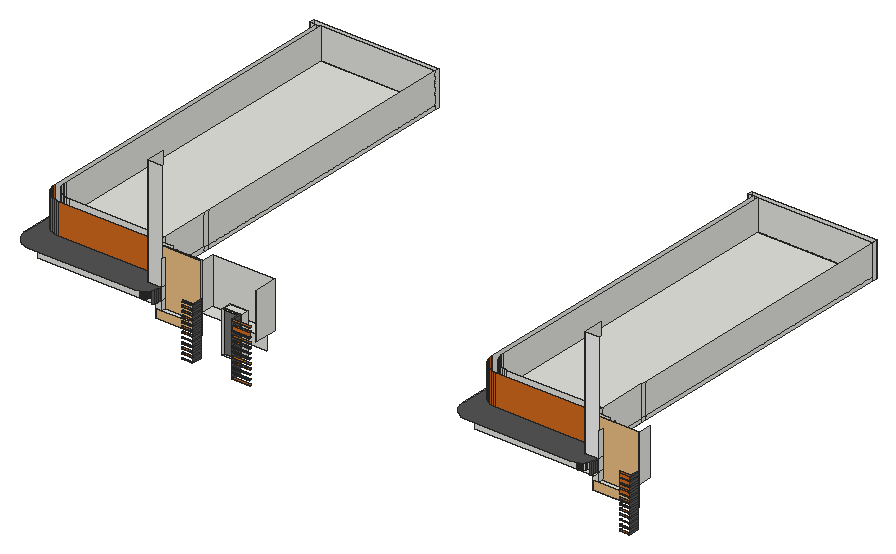
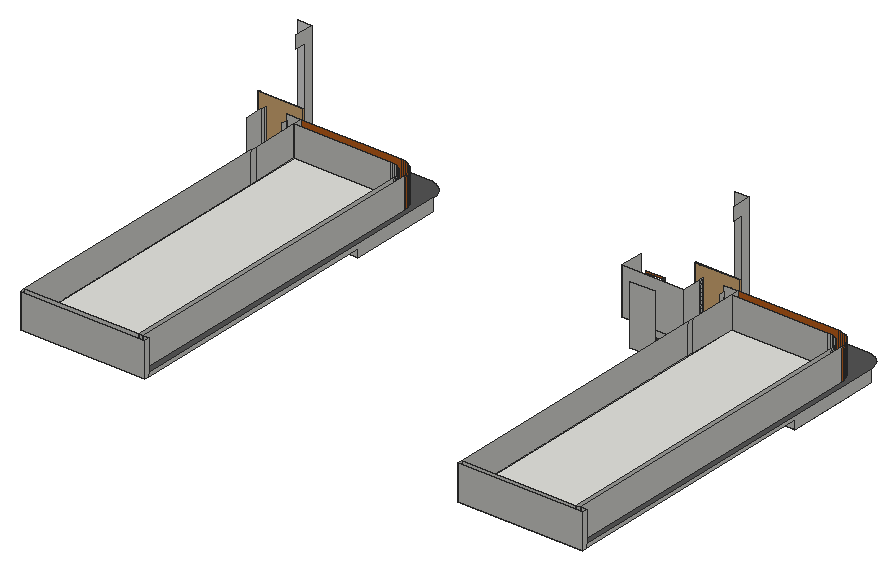
# SketchUp Ruby script. Lengths in inches.
U = 1.inch
M = Sketchup.active_model
def pt(a) = Geom::Point3d.new(a.map { |v| v * U })
def face(e, loops, mat)
  f = e.add_face(loops[0].map { |a| pt(a) })
  loops[1..].each { |l| e.add_face(l.map { |a| pt(a) }).erase! }
  f.material = f.back_material = mat if mat
  f
end
# faces: each face lists its corners as indices into pts; further lists are holes
def faces(e, pts, list, mat = nil) = list.each { |f| face(e, (f[0].is_a?(Array) ? f : [f]).map { |l| l.map { |i| pts[i] } }, mat) }
# xy, xz, yz: faces in a plane at the given z, y or x. An outline is a flat list of corners, or four numbers for a rectangle; further outlines are holes
def ring(l) = l.size == 4 ? [[l[0], l[1]], [l[2], l[1]], [l[2], l[3]], [l[0], l[3]]] : l.each_slice(2).to_a
def flat(e, list, mat, &to3) = list.each { |f| face(e, (f[0].is_a?(Array) ? f : [f]).map { |l| ring(l).map { |u, v| to3.(u, v) } }, mat) }
def xy(e, z, list, mat = nil) = flat(e, list, mat) { |x, y| [x, y, z] }
def xz(e, y, list, mat = nil) = flat(e, list, mat) { |x, z| [x, y, z] }
def yz(e, x, list, mat = nil) = flat(e, list, mat) { |y, z| [x, y, z] }
def lines(e, pts, list) = list.each { |a, b| e.add_line(pt(pts[a]), pt(pts[b])) }
# prism: a flat outline (further loops are holes) pulled along v
def prism(e, loops, v, mat = nil)
  f = face(e, loops, mat); d = Geom::Vector3d.new(v.map { |x| x * U })
  f.pushpull(f.normal.samedirection?(d) ? d.length : -d.length)
end
def box(e, o, s, mat = nil) = prism(e, [[o, [o[0] + s[0], o[1], o[2]], [o[0] + s[0], o[1] + s[1], o[2]], [o[0], o[1] + s[1], o[2]]]], [0, 0, s[2]], mat)
def at(x, y, z, deg = 0) = Geom::Transformation.translation(pt([x, y, z])) * Geom::Transformation.rotation(ORIGIN, Z_AXIS, deg.degrees)
def axes(o, x, y, z) = Geom::Transformation.new([*x, 0, *y, 0, *z, 0, *pt(o).to_a, 1])
def part(name) = M.definitions.add(name)
# library, detail: a bought-in or finely detailed component or shape, given as its bounding box
def library(name, o, s) = part(name).tap { |d| box(d.entities, o, s) }
def detail(e, o, s) = box(e.add_group.entities, o, s)
def put(e, d, t, mat = nil) = e.add_instance(d, t).tap { |i| i.material = mat if mat }
def group(e, t, mat = nil) = e.add_group.tap { |g| g.transformation = t; g.material = mat if mat }.entities
root = M.entities
M.materials.add("[0039_DarkOrange]").color = [219, 120, 0]
M.materials.add("[0041_Chocolate]").color = [210, 105, 30]
M.materials.add("[0129_WhiteSmoke]").color = [245, 245, 245]
M.materials.add("[Color M06]").color = [84, 84, 84]
M.materials.add("[Translucent Glass Gray]").color = [0, 0, 0]
M.materials["[Translucent Glass Gray]"].alpha = 0.5
c1 = library("1",[3.97,34.78,0],[101.43,33.99,0.79])
xy(root,180.58,[[820.52,971.36,835.91,972.36],[895.48,971.36,921.96,972.36],[1476.02,971.36,1491.41,972.36]],"[0041_Chocolate]")
xy(root,182.6875,[[820.52,971.36,835.91,972.36],[895.48,971.36,921.96,972.36],[1476.02,971.36,1491.41,972.36]],"[0041_Chocolate]")
xy(root,187.64,[[820.52,971.36,835.91,972.36],[895.48,971.36,921.96,972.36],[1476.02,971.36,1491.41,972.36]],"[0041_Chocolate]")
xy(root,189.75,[[820.52,971.36,835.91,972.36],[895.48,971.36,921.96,972.36],[1476.02,971.36,1491.41,972.36]],"[0041_Chocolate]")
xy(root,194.7,[[820.52,971.36,835.91,972.36],[895.48,971.36,921.96,972.36],[1476.02,971.36,1491.41,972.36]],"[0041_Chocolate]")
xy(root,196.8125,[[895.48,971.36,921.96,972.36]],"[0039_DarkOrange]")
xy(root,196.8125,[[820.52,971.36,835.91,972.36],[1476.02,971.36,1491.41,972.36]],"[0041_Chocolate]")
xy(root,196.89,[[868.14,986.55,894.83,989.22],[868.14,990.13,894.83,1001.8]])
xy(root,201.77,[[895.48,971.36,921.96,972.36]],"[0039_DarkOrange]")
xy(root,201.77,[[820.52,971.36,835.91,972.36],[1476.02,971.36,1491.41,972.36]],"[0041_Chocolate]")
xy(root,203.875,[[895.48,971.36,921.96,972.36]],"[0039_DarkOrange]")
xy(root,203.875,[[820.52,971.36,835.91,972.36],[1476.02,971.36,1491.41,972.36]],"[0041_Chocolate]")
xy(root,208.83,[[895.48,971.36,921.96,972.36]],"[0039_DarkOrange]")
xy(root,208.83,[[820.52,971.36,835.91,972.36],[1476.02,971.36,1491.41,972.36]],"[0041_Chocolate]")
xy(root,210.9375,[[895.48,971.36,921.96,972.36]],"[0039_DarkOrange]")
xy(root,210.9375,[[820.52,971.36,835.91,972.36],[1476.02,971.36,1491.41,972.36]],"[0041_Chocolate]")
xy(root,215.89,[[895.48,971.36,921.96,972.36]],"[0039_DarkOrange]")
xy(root,215.89,[[820.52,971.36,835.91,972.36],[1476.02,971.36,1491.41,972.36]],"[0041_Chocolate]")
xy(root,218,[[895.48,971.36,921.96,972.36]],"[0039_DarkOrange]")
xy(root,218,[[820.52,971.36,835.91,972.36],[1476.02,971.36,1491.41,972.36]],"[0041_Chocolate]")
xy(root,222.95,[[895.48,971.36,921.96,972.36]],"[0039_DarkOrange]")
xy(root,222.95,[[820.52,971.36,835.91,972.36],[1476.02,971.36,1491.41,972.36]],"[0041_Chocolate]")
xy(root,225.0625,[[895.48,971.36,921.96,972.36]],"[0039_DarkOrange]")
xy(root,225.0625,[[820.52,971.36,835.91,972.36],[1476.02,971.36,1491.41,972.36]],"[0041_Chocolate]")
xy(root,226.8,[[770.9,983.34,780.56,996.48],[780.56,983.34,820.52,1028.46],[1426.4,983.34,1436.06,996.48],[1436.06,983.34,1476.02,1028.46],[820.52,1008.21,913.34,1028.46]])
xy(root,227.53,[[700.74,1086.875,747.92,1094.0625],[1356.24,1086.875,1403.42,1094.0625]])
xy(root,230.02,[[895.48,971.36,921.96,972.36]],"[0039_DarkOrange]")
xy(root,230.02,[[820.52,971.36,835.91,972.36],[1476.02,971.36,1491.41,972.36]],"[0041_Chocolate]")
xy(root,232.125,[[895.48,971.36,921.96,972.36]],"[0039_DarkOrange]")
xy(root,232.125,[[820.52,971.36,835.91,972.36],[1476.02,971.36,1491.41,972.36]],"[0041_Chocolate]")
xy(root,237.08,[[895.48,971.36,921.96,972.36]],"[0039_DarkOrange]")
xy(root,237.08,[[820.52,971.36,835.91,972.36],[1476.02,971.36,1491.41,972.36]],"[0041_Chocolate]")
xy(root,239.1875,[[820.52,971.36,835.91,972.36],[895.48,971.36,921.96,972.36],[1476.02,971.36,1491.41,972.36]],"[0041_Chocolate]")
xy(root,240.16,[[756.44,972.36,757.68,972.44,758.91,972.69,759.32,972.82,759.32,972.36],[759.32,972.36,759.32,972.82,760.09,973.09,761.21,973.64,762.24,974.33,763.18,975.15,764,976.09,764.7,977.13,765.25,978.25,765.65,979.43,765.89,980.65,765.97,981.89,759.32,981.89,759.32,983.34,779.69,983.34,779.69,981.89,779.49,978.86,778.9,975.875,777.92,973,777.61,972.36],[777.61,972.36,780.56,972.36,780.56,981.89,779.69,981.89,779.49,978.86,778.9,975.875,777.92,973],[1411.94,972.36,1413.18,972.44,1414.41,972.69,1414.82,972.82,1414.82,972.36],[1414.82,972.36,1414.82,972.82,1415.59,973.09,1416.71,973.64,1417.74,974.33,1418.68,975.15,1419.5,976.09,1420.2,977.13,1420.75,978.25,1421.15,979.43,1421.39,980.65,1421.47,981.89,1414.82,981.89,1414.82,983.34,1435.19,983.34,1435.19,981.89,1434.99,978.86,1434.4,975.875,1433.42,973,1433.11,972.36],
  [1433.11,972.36,1436.06,972.36,1436.06,981.89,1435.19,981.89,1434.99,978.86,1434.4,975.875,1433.42,973],[759.32,972.82,760.09,973.09,761.21,973.64,762.24,974.33,763.18,975.15,764,976.09,764.7,977.13,765.25,978.25,765.65,979.43,765.89,980.65,765.97,981.89,759.32,981.89],[1414.82,972.82,1415.59,973.09,1416.71,973.64,1417.74,974.33,1418.68,975.15,1419.5,976.09,1420.2,977.13,1420.75,978.25,1421.15,979.43,1421.39,980.65,1421.47,981.89,1414.82,981.89],[779.69,981.89,780.56,983.34],[1435.19,981.89,1436.06,983.34],
  [759.32,983.34,779.69,1003.71],[779.69,983.34,780.56,1003.71],[1414.82,983.34,1435.19,1003.71],[1435.19,983.34,1436.06,1003.71]])
xy(root,240.16,[[572.21,1024.22,585.93,1130.875],[1227.71,1024.22,1241.43,1130.875]],"[Color M06]")
xy(root,244.14,[[820.52,971.36,835.91,972.36],[895.48,971.36,921.96,972.36],[1476.02,971.36,1491.41,972.36]],"[0041_Chocolate]")
xy(root,246.25,[[820.52,971.36,835.91,972.36],[895.48,971.36,921.96,972.36],[1476.02,971.36,1491.41,972.36]],"[0041_Chocolate]")
xy(root,251.2,[[820.52,971.36,835.91,972.36],[895.48,971.36,921.96,972.36],[1476.02,971.36,1491.41,972.36]],"[0041_Chocolate]")
xy(root,252.47,[[602.85,972.36,600.64,972.5,598.47,972.9375,596.37,973.65,594.39,974.63,592.55,975.86,590.88,977.32,589.42,978.98,588.19,980.82,587.21,982.81,586.5,984.9,586.07,987.07,585.93,989.28,585.93,1130.875,688.99,1130.875,688.99,1086.875,759.32,1086.875,759.32,981.89,765.97,981.89,765.89,980.65,765.65,979.43,765.25,978.25,764.7,977.13,764,976.09,763.18,975.15,762.24,974.33,761.21,973.64,760.09,973.09,758.91,972.69,757.68,972.44,756.44,972.36],[1258.35,972.36,1256.14,972.5,1253.97,972.9375,1251.87,973.65,1249.89,974.63,1248.05,975.86,1246.38,977.32,1244.92,978.98,1243.69,980.82,1242.71,982.81,1242,984.9,1241.57,987.07,1241.43,989.28,1241.43,1130.875,1344.49,1130.875,1344.49,1086.875,1414.82,1086.875,1414.82,981.89,1421.47,981.89,1421.39,980.65,1421.15,979.43,1420.75,978.25,1420.2,977.13,1419.5,976.09,1418.68,975.15,1417.74,974.33,1416.71,973.64,1415.59,973.09,1414.41,972.69,1413.18,972.44,1411.94,972.36],[[688.99,1086.875,759.32,1086.875,759.32,1094.0625,706.57,1094.0625,706.57,1130.875,759.32,1130.875,759.32,1521.81,572.21,1521.81,572.21,1130.875,688.99,1130.875],[577.71,1136.38,753.81,1516.3]],[[1344.49,1086.875,1414.82,1086.875,1414.82,1094.0625,1362.07,1094.0625,1362.07,1130.875,1414.82,1130.875,1414.82,1521.81,1227.71,1521.81,1227.71,1130.875,1344.49,1130.875],[1233.21,1136.38,1409.31,1516.3]],[706.57,1094.0625,759.32,1130.875],
  [1362.07,1094.0625,1414.82,1130.875],[572.21,1521.81,759.32,1529.04],[1227.71,1521.81,1414.82,1529.04]])
xy(root,253.3125,[[820.52,971.36,835.91,972.36],[895.48,971.36,921.96,972.36],[1476.02,971.36,1491.41,972.36]],"[0041_Chocolate]")
xy(root,258.13,[[779.69,983.34,780.56,1003.71],[1435.19,983.34,1436.06,1003.71],[615.56,1016.23,759.32,1016.23,759.32,1521.81,587.54,1521.81,587.54,1044.25,587.78,1040.6,588.49,1037,589.67,1033.53,591.29,1030.24,593.33,1027.2,595.74,1024.44,598.5,1022.02,601.55,1019.99,604.83,1018.37,608.31,1017.1875,611.9,1016.47],[1271.06,1016.23,1414.82,1016.23,1414.82,1521.81,1243.04,1521.81,1243.04,1044.25,1243.28,1040.6,1243.99,1037,1245.17,1033.53,1246.79,1030.24,1248.83,1027.2,1251.24,1024.44,1254,1022.02,1257.05,1019.99,1260.33,1018.37,1263.81,1017.1875,1267.4,1016.47]])
xy(root,258.13,[[602.85,958.64,756.44,958.64,759.48,958.84,762.46,959.4375,765.34,960.41,768.07,961.76,770.59,963.45,772.88,965.45,774.89,967.74,776.58,970.27,777.92,973,778.9,975.875,779.49,978.86,779.69,981.89,779.69,1003.71,609.8125,1003.71,606.02,1003.96,602.29,1004.7,598.69,1005.92,595.28,1007.6,592.12,1009.71,589.26,1012.22,586.76,1015.08,585.98,1016.23,584.65,1018.24,582.96,1021.65,581.74,1025.25,581,1028.97,580.75,1032.77,580.75,1521.81,572.21,1521.81,572.21,989.28,572.47,985.28,573.25,981.35,574.54,977.56,576.3125,973.96,578.54,970.63,581.18,967.62,584.2,964.98,587.53,962.75,591.125,960.98,594.92,959.6875,598.85,958.91],[1258.35,958.64,1411.94,958.64,1414.98,958.84,1417.96,959.4375,1420.84,960.41,1423.57,961.76,1426.09,963.45,1428.38,965.45,1430.39,967.74,1432.08,970.27,1433.42,973,1434.4,975.875,1434.99,978.86,1435.19,981.89,1435.19,1003.71,1265.3125,1003.71,1261.52,1003.96,1257.79,1004.7,1254.19,1005.92,1250.78,1007.6,1247.62,1009.71,1244.76,1012.22,1242.26,1015.08,1241.48,1016.23,1240.15,1018.24,1238.46,1021.65,1237.24,1025.25,1236.5,1028.97,1236.25,1032.77,1236.25,1521.81,1227.71,1521.81,1227.71,989.28,1227.97,985.28,1228.75,981.35,1230.04,977.56,1231.8125,973.96,1234.04,970.63,1236.68,967.62,1239.7,964.98,1243.03,962.75,1246.625,960.98,1250.42,959.6875,1254.35,958.91]],"[Color M06]")
xy(root,258.27,[[868.14,986.55,894.83,989.22],[868.14,989.22,894.83,990.13],[868.14,990.13,894.83,1001.8]])
xy(root,258.27,[[820.52,971.36,836.56,972.36],[894.83,971.36,921.96,972.36],[1476.02,971.36,1492.06,972.36]],"[0041_Chocolate]")
xz(root,971.36,[[1476.02,232.125,1491.41,237.08],[1476.02,239.1875,1491.41,244.14],[895.48,246.25,921.96,251.2],[1476.02,246.25,1491.41,251.2],[1476.02,253.3125,1491.41,253.3125,1492.06,258.27,1476.02,258.27]],"[0041_Chocolate]")
xz(root,972.36,[[602.85,240.16,756.44,252.47],[1258.35,240.16,1411.94,252.47]])
xz(root,972.36,[[895.48,201.77,921.96,203.875],[895.48,208.83,921.96,210.9375],[895.48,215.89,921.96,218],[895.48,222.95,921.96,225.0625],[895.48,230.02,921.96,232.125],
  [895.48,237.08,921.96,239.1875]],"[0039_DarkOrange]")
xz(root,972.36,[[820.52,180.58,835.91,182.6875],[895.48,180.58,921.96,182.6875],[1476.02,180.58,1491.41,182.6875],[820.52,187.64,835.91,189.75],[895.48,187.64,921.96,189.75],
  [1476.02,187.64,1491.41,189.75],[820.52,194.7,835.91,196.8125],[895.48,194.7,921.96,196.8125],[1476.02,194.7,1491.41,196.8125],[820.52,201.77,835.91,203.875],
  [1476.02,201.77,1491.41,203.875],[820.52,208.83,835.91,210.9375],[1476.02,208.83,1491.41,210.9375],[820.52,215.89,835.91,218],[1476.02,215.89,1491.41,218],
  [820.52,222.95,835.91,225.0625],[1476.02,222.95,1491.41,225.0625],[820.52,230.02,835.91,232.125],[1476.02,230.02,1491.41,232.125],[820.52,237.08,835.91,239.1875],
  [1476.02,237.08,1491.41,239.1875],[820.52,244.14,835.91,246.25],[895.48,244.14,921.96,246.25],[1476.02,244.14,1491.41,246.25],[820.52,251.2,835.91,253.3125],
  [895.48,251.2,921.96,253.3125],[1476.02,251.2,1491.41,253.3125],[820.52,258.27,836.56,258.27,836.84,260.375,820.52,260.375],[894.83,258.27,921.96,258.27,921.96,260.375,894.55,260.375],[1476.02,258.27,1492.06,258.27,1492.34,260.375,1476.02,260.375]],"[0041_Chocolate]")
xz(root,981.89,[[759.32,240.16,765.97,252.47],[1414.82,240.16,1421.47,252.47]])
xz(root,983.34,[[770.9,226.8,780.56,240.16],[1426.4,226.8,1436.06,240.16],[759.32,240.16,779.69,240.16,779.69,258.13,780.56,258.13,780.56,421.25,759.32,421.25],[779.69,240.16,780.56,258.13],[1435.19,240.16,1436.06,258.13]])
xz(root,983.34,[[1414.82,240.16,1435.19,240.16,1435.19,258.13,1436.06,258.13,1436.06,421.25,1414.82,421.25]],"[0129_WhiteSmoke]")
xz(root,989.22,[[868.14,196.89,894.83,258.27]],"[Translucent Glass Gray]")
xz(root,990.13,[[868.14,196.89,894.83,258.27]])
xz(root,1001.8,[[868.14,196.89,894.83,258.27]])
xz(root,1003.71,[[759.32,240.16,779.69,258.13],[779.69,240.16,780.56,258.13],[1414.82,240.16,1435.19,258.13],[1435.19,240.16,1436.06,258.13],[759.32,258.13,780.56,304.25],
  [1414.82,258.13,1436.06,304.25]])
xz(root,1003.71,[[609.8125,258.13,759.32,304.25],[1265.3125,258.13,1414.82,304.25]],"[0041_Chocolate]")
xz(root,1016.23,[[615.56,258.13,759.32,304.25],[1271.06,258.13,1414.82,304.25]])
xz(root,1028.46,[[820.52,226.8,913.34,295.72]])
xz(root,1032.54,[[860.9,192.35,897.76,281.26]])
xz(root,1130.875,[[572.21,240.16,585.93,252.47],[1227.71,240.16,1241.43,252.47]])
xz(root,1521.81,[[572.21,252.47,572.21,258.13,580.75,258.13,580.75,304.25,587.54,304.25,587.54,258.13,759.32,258.13,759.32,252.47],[1227.71,252.47,1227.71,258.13,1236.25,258.13,1236.25,304.25,1243.04,304.25,1243.04,258.13,1414.82,258.13,1414.82,252.47],[572.21,258.13,580.75,304.25],[587.54,258.13,759.32,304.25],[1227.71,258.13,1236.25,304.25],
  [1243.04,258.13,1414.82,304.25]])
xz(root,1529.04,[[572.21,252.47,759.32,304.25],[1227.71,252.47,1414.82,304.25]])
yz(root,572.21,[[989.28,240.16,989.28,258.13,1521.81,258.13,1521.81,252.47,1130.875,252.47,1130.875,240.16],[1521.81,252.47,1529.04,304.25]])
yz(root,580.75,[[1032.77,258.13,1521.81,304.25]])
yz(root,585.93,[[989.28,240.16,1130.875,252.47]],"[Color M06]")
yz(root,587.54,[[1044.25,258.13,1521.81,304.25]])
yz(root,759.32,[[981.89,240.16,983.34,252.47],[983.34,240.16,996.48,252.47],[996.48,240.16,1003.71,252.47],[983.34,252.47,983.34,421.25,1012.23,421.25,1012.23,402.64,996.48,402.64,996.48,252.47],[1003.71,252.47,1088.75,252.47,1088.75,258.13,1016.23,258.13,1016.23,304.25,1003.71,304.25],
  [1088.75,252.47,1097.28,258.13],[1097.28,252.47,1521.81,258.13],[1521.81,252.47,1529.04,304.25],[1016.23,258.13,1088.75,304.25],[1088.75,258.13,1097.28,304.25],
  [1097.28,258.13,1521.81,304.25]])
yz(root,779.69,[[981.89,240.16,983.34,258.13],[983.34,240.16,1003.71,258.13]])
yz(root,780.56,[[983.34,226.8,996.48,240.16],[996.48,226.8,1012.23,240.16],[1012.23,226.8,1028.46,240.16],[983.34,240.16,996.48,258.13],[1003.71,240.16,1012.23,258.13],
  [1012.23,240.16,1028.46,258.13],[983.34,258.13,996.48,295.72],[996.48,258.13,1003.71,295.72],[1003.71,258.13,1012.23,295.72]])
yz(root,820.52,[[992.96,226.8,993.35,295.72],[993.35,226.8,996.48,295.72],[996.48,226.8,1001.16,295.72],[1001.16,226.8,1028.46,295.72]])
yz(root,835.91,[[972.36,180.58,986.55,182.6875],[971.36,182.6875,986.55,187.64],[972.36,187.64,986.55,189.75],[971.36,189.75,986.55,194.7],[972.36,194.7,986.55,196.8125],
  [971.36,196.8125,986.55,201.77],[972.36,201.77,986.55,203.875],[971.36,203.875,986.55,208.83],[972.36,208.83,986.55,210.9375],[971.36,210.9375,986.55,215.89],
  [972.36,215.89,986.55,218],[971.36,218,986.55,222.95],[972.36,222.95,986.55,225.0625],[971.36,225.0625,986.55,230.02],[972.36,230.02,986.55,232.125],
  [971.36,232.125,986.55,237.08],[972.36,237.08,986.55,239.1875],[971.36,239.1875,986.55,244.14],[972.36,244.14,986.55,246.25],[971.36,246.25,986.55,251.2],
  [972.36,251.2,986.55,253.3125]],"[Color M06]")
yz(root,868.14,[[986.55,196.89,989.22,258.27],[990.13,196.89,1001.8,258.27]])
yz(root,894.83,[[986.55,196.89,989.22,258.27],[990.13,196.89,1001.8,258.27]])
yz(root,895.48,[[972.36,180.58,986.55,182.6875],[971.36,182.6875,986.55,187.64],[972.36,187.64,986.55,189.75],[971.36,189.75,986.55,194.7],[972.36,194.7,986.55,196.8125],
  [971.36,196.8125,986.55,201.77],[972.36,201.77,986.55,203.875],[971.36,203.875,986.55,208.83],[972.36,208.83,986.55,210.9375],[971.36,210.9375,986.55,215.89],
  [972.36,215.89,986.55,218],[971.36,218,986.55,222.95],[972.36,222.95,986.55,225.0625],[971.36,225.0625,986.55,230.02],[972.36,230.02,986.55,232.125],
  [971.36,232.125,986.55,237.08],[972.36,237.08,986.55,239.1875],[971.36,239.1875,986.55,244.14],[972.36,244.14,986.55,246.25],[971.36,246.25,986.55,251.2],
  [972.36,251.2,986.55,253.3125]],"[Color M06]")
yz(root,913.34,[[992.96,226.8,993.35,295.72],[993.35,226.8,1028.46,295.72]])
yz(root,1227.71,[[989.28,240.16,989.28,258.13,1521.81,258.13,1521.81,252.47,1130.875,252.47,1130.875,240.16],[1521.81,252.47,1529.04,304.25]])
yz(root,1236.25,[[1032.77,258.13,1521.81,304.25]])
yz(root,1241.43,[[989.28,240.16,1130.875,252.47]],"[Color M06]")
yz(root,1243.04,[[1044.25,258.13,1521.81,304.25]])
yz(root,1414.82,[[981.89,240.16,983.34,252.47],[983.34,240.16,996.48,252.47],[996.48,240.16,1003.71,252.47],[983.34,252.47,983.34,421.25,1012.23,421.25,1012.23,402.64,996.48,402.64,996.48,252.47],[1003.71,252.47,1088.75,252.47,1088.75,258.13,1016.23,258.13,1016.23,304.25,1003.71,304.25],
  [1088.75,252.47,1097.28,258.13],[1097.28,252.47,1521.81,258.13],[1521.81,252.47,1529.04,304.25],[1016.23,258.13,1088.75,304.25],[1088.75,258.13,1097.28,304.25],
  [1097.28,258.13,1521.81,304.25]])
yz(root,1435.19,[[981.89,240.16,983.34,258.13],[983.34,240.16,1003.71,258.13]])
yz(root,1436.06,[[983.34,226.8,996.48,240.16],[996.48,226.8,1012.23,240.16],[1012.23,226.8,1028.46,240.16],[983.34,240.16,996.48,258.13],[1003.71,240.16,1012.23,258.13],
  [1012.23,240.16,1028.46,258.13],[983.34,258.13,996.48,295.72],[996.48,258.13,1003.71,295.72],[1003.71,258.13,1012.23,295.72]])
yz(root,1476.02,[[992.96,226.8,993.35,295.72],[993.35,226.8,996.48,295.72],[996.48,226.8,1001.16,295.72],[1001.16,226.8,1028.46,295.72]])
yz(root,1491.41,[[972.36,180.58,986.55,182.6875],[971.36,182.6875,986.55,187.64],[972.36,187.64,986.55,189.75],[971.36,189.75,986.55,194.7],[972.36,194.7,986.55,196.8125],
  [971.36,196.8125,986.55,201.77],[972.36,201.77,986.55,203.875],[971.36,203.875,986.55,208.83],[972.36,208.83,986.55,210.9375],[971.36,210.9375,986.55,215.89],
  [972.36,215.89,986.55,218],[971.36,218,986.55,222.95],[972.36,222.95,986.55,225.0625],[971.36,225.0625,986.55,230.02],[972.36,230.02,986.55,232.125],
  [971.36,232.125,986.55,237.08],[972.36,237.08,986.55,239.1875],[971.36,239.1875,986.55,244.14],[972.36,244.14,986.55,246.25],[971.36,246.25,986.55,251.2],
  [972.36,251.2,986.55,253.3125]],"[Color M06]")
p = [[777.92,973,258.13],[776.58,970.27,258.13],[776.58,970.27,240.16],[777.61,972.36,240.16],[777.92,973,240.16],[1433.42,973,258.13],
  [1432.08,970.27,258.13],[1432.08,970.27,240.16],[1433.11,972.36,240.16],[1433.42,973,240.16],[756.44,972.36,252.47],[757.68,972.44,252.47],
  [757.68,972.44,240.16],[756.44,972.36,240.16],[758.91,972.69,252.47],[758.91,972.69,240.16],[1411.94,972.36,252.47],[1413.18,972.44,252.47],
  [1413.18,972.44,240.16],[1411.94,972.36,240.16],[1414.41,972.69,252.47],[1414.41,972.69,240.16],[760.09,973.09,252.47],[760.09,973.09,240.16],
  [759.32,972.82,240.16],[1415.59,973.09,252.47],[1415.59,973.09,240.16],[1414.82,972.82,240.16],[778.9,975.875,258.13],[778.9,975.875,240.16],
  [1434.4,975.875,258.13],[1434.4,975.875,240.16],[761.21,973.64,252.47],[761.21,973.64,240.16],[1416.71,973.64,252.47],[1416.71,973.64,240.16],
  [762.24,974.33,252.47],[762.24,974.33,240.16],[1417.74,974.33,252.47],[1417.74,974.33,240.16],[763.18,975.15,252.47],[763.18,975.15,240.16],
  [1418.68,975.15,252.47],[1418.68,975.15,240.16],[764,976.09,252.47],[764,976.09,240.16],[1419.5,976.09,252.47],[1419.5,976.09,240.16],
  [779.49,978.86,258.13],[779.49,978.86,240.16],[1434.99,978.86,258.13],[1434.99,978.86,240.16],[764.7,977.13,252.47],[764.7,977.13,240.16],
  [1420.2,977.13,252.47],[1420.2,977.13,240.16],[765.25,978.25,252.47],[765.25,978.25,240.16],[1420.75,978.25,252.47],[1420.75,978.25,240.16],
  [765.65,979.43,252.47],[765.65,979.43,240.16],[1421.15,979.43,252.47],[1421.15,979.43,240.16],[779.69,981.89,258.13],[779.69,981.89,240.16],
  [1435.19,981.89,258.13],[1435.19,981.89,240.16],[765.89,980.65,252.47],[765.89,980.65,240.16],[1421.39,980.65,252.47],[1421.39,980.65,240.16],
  [765.97,981.89,252.47],[765.97,981.89,240.16],[1421.47,981.89,252.47],[1421.47,981.89,240.16],[836.56,986.55,258.27],[836.56,972.36,258.27],
  [836.56,971.36,258.27],[835.91,971.36,253.3125],[835.91,972.36,253.3125],[835.91,986.55,253.3125],[895.48,986.55,253.3125],[895.48,972.36,253.3125],
  [895.48,971.36,253.3125],[894.83,971.36,258.27],[894.83,972.36,258.27],[894.83,986.55,258.27],[1492.06,986.55,258.27],[1492.06,972.36,258.27],
  [1492.06,971.36,258.27],[1491.41,971.36,253.3125],[1491.41,972.36,253.3125],[1491.41,986.55,253.3125],[606.02,1003.96,258.13],[609.8125,1003.71,258.13],
  [609.8125,1003.71,304.25],[606.02,1003.96,304.25],[1261.52,1003.96,258.13],[1265.3125,1003.71,258.13],[1265.3125,1003.71,304.25],[1261.52,1003.96,304.25],
  [602.29,1004.7,258.13],[602.29,1004.7,304.25],[1257.79,1004.7,258.13],[1257.79,1004.7,304.25],[598.69,1005.92,258.13],[598.69,1005.92,304.25],
  [1254.19,1005.92,258.13],[1254.19,1005.92,304.25],[595.28,1007.6,258.13],[595.28,1007.6,304.25],[1250.78,1007.6,258.13],[1250.78,1007.6,304.25],
  [592.12,1009.71,258.13],[592.12,1009.71,304.25],[1247.62,1009.71,258.13],[1247.62,1009.71,304.25],[589.26,1012.22,258.13],[589.26,1012.22,304.25],
  [1244.76,1012.22,258.13],[1244.76,1012.22,304.25],[586.76,1015.08,258.13],[587.54,1014.1875,304.25],[586.76,1015.08,304.25],[1242.26,1015.08,258.13],
  [1243.04,1014.1875,304.25],[1242.26,1015.08,304.25],[585.98,1016.23,258.13],[585.98,1016.23,304.25],[1241.48,1016.23,258.13],[1241.48,1016.23,304.25],
  [584.65,1018.24,258.13],[584.65,1018.24,304.25],[615.56,1016.23,258.13],[611.9,1016.47,258.13],[611.9,1016.47,304.25],[615.56,1016.23,304.25],
  [1240.15,1018.24,258.13],[1240.15,1018.24,304.25],[1271.06,1016.23,258.13],[1267.4,1016.47,258.13],[1267.4,1016.47,304.25],[1271.06,1016.23,304.25],
  [608.31,1017.1875,258.13],[608.31,1017.1875,304.25],[1263.81,1017.1875,258.13],[1263.81,1017.1875,304.25],[604.83,1018.37,258.13],[604.83,1018.37,304.25],
  [1260.33,1018.37,258.13],[1260.33,1018.37,304.25],[582.96,1021.65,258.13],[582.96,1021.65,304.25],[1238.46,1021.65,258.13],[1238.46,1021.65,304.25],
  [601.55,1019.99,258.13],[601.55,1019.99,304.25],[1257.05,1019.99,258.13],[1257.05,1019.99,304.25],[598.5,1022.02,258.13],[598.5,1022.02,304.25],
  [1254,1022.02,258.13],[1254,1022.02,304.25],[581.74,1025.25,258.13],[581.74,1025.25,304.25],[1237.24,1025.25,258.13],[1237.24,1025.25,304.25],
  [595.74,1024.44,258.13],[595.74,1024.44,304.25],[1251.24,1024.44,258.13],[1251.24,1024.44,304.25],[593.33,1027.2,258.13],[593.33,1027.2,304.25],
  [1248.83,1027.2,258.13],[1248.83,1027.2,304.25],[581,1028.97,258.13],[581,1028.97,304.25],[1236.5,1028.97,258.13],[1236.5,1028.97,304.25],
  [591.29,1030.24,258.13],[591.29,1030.24,304.25],[1246.79,1030.24,258.13],[1246.79,1030.24,304.25],[580.75,1032.77,258.13],[580.75,1032.77,304.25],
  [1236.25,1032.77,258.13],[1236.25,1032.77,304.25],[589.67,1033.53,258.13],[589.67,1033.53,304.25],[1245.17,1033.53,258.13],[1245.17,1033.53,304.25],
  [588.49,1037,258.13],[588.49,1037,304.25],[1243.99,1037,258.13],[1243.99,1037,304.25],[587.78,1040.6,258.13],[587.78,1040.6,304.25],
  [1243.28,1040.6,258.13],[1243.28,1040.6,304.25],[587.54,1044.25,258.13],[587.54,1044.25,304.25],[1243.04,1044.25,258.13],[1243.04,1044.25,304.25],
  [836.84,972.36,260.375],[836.84,986.55,260.375],[894.55,972.36,260.375],[894.55,986.55,260.375],[1492.34,972.36,260.375],[1492.34,986.55,260.375],
  [860.9,1012.23,192.35],[860.9,1032.54,192.35]]
faces(root,p,[[0,1,2,3,4],[5,6,7,8,9],[28,0,4,29],[30,5,9,31],[48,28,29,49],[50,30,31,51],[64,48,49,65],[66,50,51,67],
  [76,77,78,79,80,81],[82,83,84,85,86,87],[88,89,90,91,92,93],[204,77,76,205],[86,206,207,87],[208,89,88,209]],"[Color M06]")
faces(root,p,[[10,11,12,13],[11,14,15,12],[16,17,18,19],[17,20,21,18],[14,22,23,24,15],[20,25,26,27,21],[22,32,33,23],[25,34,35,26],
  [32,36,37,33],[34,38,39,35],[36,40,41,37],[38,42,43,39],[40,44,45,41],[42,46,47,43],[44,52,53,45],[46,54,55,47],
  [52,56,57,53],[54,58,59,55],[56,60,61,57],[58,62,63,59],[60,68,69,61],[62,70,71,63],[68,72,73,69],[70,74,75,71],
  [134,135,136,137],[140,141,142,143],[135,144,145,136],[141,146,147,142],[144,148,149,145],[146,150,151,147],[148,156,157,149],[150,158,159,151],
  [156,160,161,157],[158,162,163,159],[160,168,169,161],[162,170,171,163],[168,172,173,169],[170,174,175,171],[172,180,181,173],[174,182,183,175],
  [180,188,189,181],[182,190,191,183],[188,192,193,189],[190,194,195,191],[192,196,197,193],[194,198,199,195],[196,200,201,197],[198,202,203,199]])
faces(root,p,[[94,95,96,97],[98,99,100,101],[102,94,97,103],[104,98,101,105],[106,102,103,107],[108,104,105,109],[110,106,107,111],[112,108,109,113],
  [114,110,111,115],[116,112,113,117],[118,114,115,119],[120,116,117,121],[122,118,119,123,124],[125,120,121,126,127],[128,122,124,129],[130,125,127,131],
  [132,128,129,133],[138,130,131,139],[152,132,133,153],[154,138,139,155],[164,152,153,165],[166,154,155,167],[176,164,165,177],[178,166,167,179],
  [184,176,177,185],[186,178,179,187]],"[0041_Chocolate]")
lines(root,p,[[210,211]])
put(root,c1,axes([904.18,990.33,204.87],[0,0,1],[-2,0,0],[0,-1,0]))
put(root,c1,axes([1559.68,990.33,204.87],[0,0,1],[-2,0,0],[0,-1,0]))
